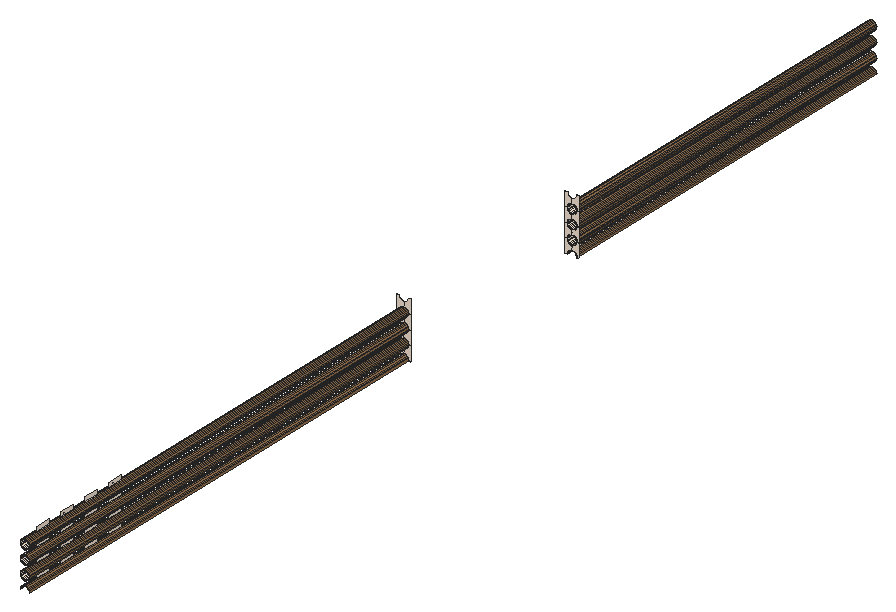
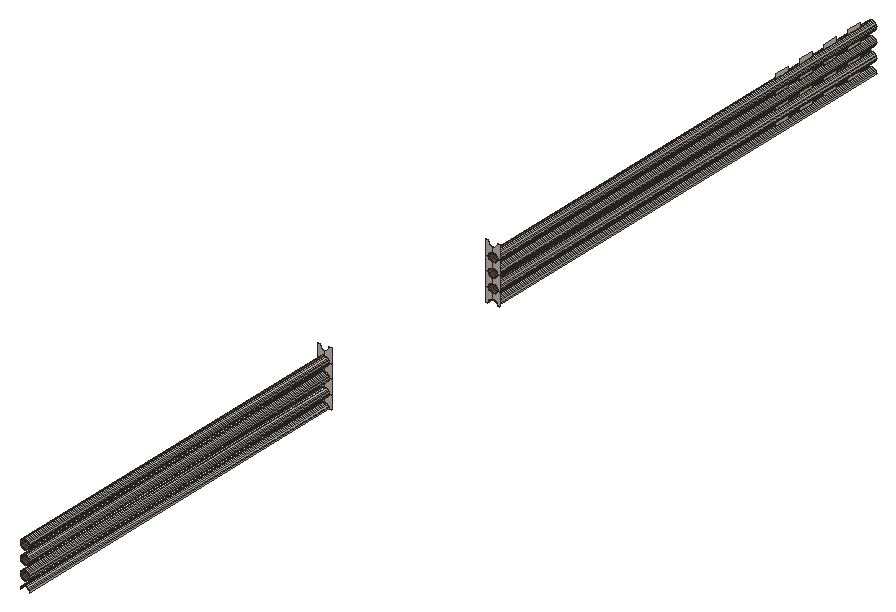
# SketchUp Ruby script. Lengths in inches.
U = 1.inch
M = Sketchup.active_model
def pt(a) = Geom::Point3d.new(a.map { |v| v * U })
def face(e, loops, mat)
  f = e.add_face(loops[0].map { |a| pt(a) })
  loops[1..].each { |l| e.add_face(l.map { |a| pt(a) }).erase! }
  f.material = f.back_material = mat if mat
  f
end
# faces: each face lists its corners as indices into pts; further lists are holes
def faces(e, pts, list, mat = nil) = list.each { |f| face(e, (f[0].is_a?(Array) ? f : [f]).map { |l| l.map { |i| pts[i] } }, mat) }
# xy, xz, yz: faces in a plane at the given z, y or x. An outline is a flat list of corners, or four numbers for a rectangle; further outlines are holes
def ring(l) = l.size == 4 ? [[l[0], l[1]], [l[2], l[1]], [l[2], l[3]], [l[0], l[3]]] : l.each_slice(2).to_a
def flat(e, list, mat, &to3) = list.each { |f| face(e, (f[0].is_a?(Array) ? f : [f]).map { |l| ring(l).map { |u, v| to3.(u, v) } }, mat) }
def xy(e, z, list, mat = nil) = flat(e, list, mat) { |x, y| [x, y, z] }
def xz(e, y, list, mat = nil) = flat(e, list, mat) { |x, z| [x, y, z] }
def yz(e, x, list, mat = nil) = flat(e, list, mat) { |y, z| [x, y, z] }
def lines(e, pts, list) = list.each { |a, b| e.add_line(pt(pts[a]), pt(pts[b])) }
# prism: a flat outline (further loops are holes) pulled along v
def prism(e, loops, v, mat = nil)
  f = face(e, loops, mat); d = Geom::Vector3d.new(v.map { |x| x * U })
  f.pushpull(f.normal.samedirection?(d) ? d.length : -d.length)
end
def box(e, o, s, mat = nil) = prism(e, [[o, [o[0] + s[0], o[1], o[2]], [o[0] + s[0], o[1] + s[1], o[2]], [o[0], o[1] + s[1], o[2]]]], [0, 0, s[2]], mat)
def at(x, y, z, deg = 0) = Geom::Transformation.translation(pt([x, y, z])) * Geom::Transformation.rotation(ORIGIN, Z_AXIS, deg.degrees)
def axes(o, x, y, z) = Geom::Transformation.new([*x, 0, *y, 0, *z, 0, *pt(o).to_a, 1])
def part(name) = M.definitions.add(name)
# library, detail: a bought-in or finely detailed component or shape, given as its bounding box
def library(name, o, s) = part(name).tap { |d| box(d.entities, o, s) }
def detail(e, o, s) = box(e.add_group.entities, o, s)
def put(e, d, t, mat = nil) = e.add_instance(d, t).tap { |i| i.material = mat if mat }
def group(e, t, mat = nil) = e.add_group.tap { |g| g.transformation = t; g.material = mat if mat }.entities
root = M.entities
M.materials.add("C01_Vanilla_Cream").color = [244, 228, 212]
M.materials.add("Wood_Floor_01_1K").color = [146, 111, 76]
xz(root,216,[[354,168,355,168,355.07,168.52,355.27,169,355.59,169.41,356,169.73,356.48,169.93,357,170,357,172,356.48,172.07,356,172.27,355.59,172.59,355.27,173,355.07,173.48,355,174,354,174],[359,168,360,168,360,174,359,174,358.93,173.48,358.73,173,358.41,172.59,358,172.27,357.52,172.07,357,172,357,170,357.52,169.93,358,169.73,358.41,169.41,358.73,169,358.93,168.52],[354,174,355,174,355.07,174.52,355.27,175,355.59,175.41,356,175.73,356.48,175.93,357,176,357,178,356.48,178.07,356,178.27,355.59,178.59,355.27,179,355.07,179.48,355,180,354,180],[359,174,360,174,360,180,359,180,358.93,179.48,358.73,179,358.41,178.59,358,178.27,357.52,178.07,357,178,357,176,357.52,175.93,358,175.73,358.41,175.41,358.73,175,358.93,174.52],[354,180,355,180,355.07,180.52,355.27,181,355.59,181.41,356,181.73,356.48,181.93,357,182,357,184,356.48,184.07,356,184.27,355.59,184.59,355.27,185,355.07,185.48,355,186,354,186],
  [359,180,360,180,360,186,359,186,358.93,185.48,358.73,185,358.41,184.59,358,184.27,357.52,184.07,357,184,357,182,357.52,181.93,358,181.73,358.41,181.41,358.73,181,358.93,180.52],[354,186,355,186,355.07,186.52,355.27,187,355.59,187.41,356,187.73,356.48,187.93,357,188,357,190,356.48,190.07,356,190.27,355.59,190.59,355.27,191,355.07,191.48,355,192,354,192],[359,186,360,186,360,192,359,192,358.93,191.48,358.73,191,358.41,190.59,358,190.27,357.52,190.07,357,190,357,188,357.52,187.93,358,187.73,358.41,187.41,358.73,187,358.93,186.52]],"C01_Vanilla_Cream")
xz(root,306.76,[[354,168,354,174,355,174,355.07,173.48,355.27,173,355.59,172.59,356,172.27,356.48,172.07,357,172,357,170,356.48,169.93,356,169.73,355.59,169.41,355.27,169,355.07,168.52,355,168],[359,168,358.93,168.52,358.73,169,358.41,169.41,358,169.73,357.52,169.93,357,170,357,172,357.52,172.07,358,172.27,358.41,172.59,358.73,173,358.93,173.48,359,174,360,174,360,168],[354,174,354,180,355,180,355.07,179.48,355.27,179,355.59,178.59,356,178.27,356.48,178.07,357,178,357,176,356.48,175.93,356,175.73,355.59,175.41,355.27,175,355.07,174.52,355,174],[359,174,358.93,174.52,358.73,175,358.41,175.41,358,175.73,357.52,175.93,357,176,357,178,357.52,178.07,358,178.27,358.41,178.59,358.73,179,358.93,179.48,359,180,360,180,360,174],[354,180,354,186,355,186,355.07,185.48,355.27,185,355.59,184.59,356,184.27,356.48,184.07,357,184,357,182,356.48,181.93,356,181.73,355.59,181.41,355.27,181,355.07,180.52,355,180],
  [359,180,358.93,180.52,358.73,181,358.41,181.41,358,181.73,357.52,181.93,357,182,357,184,357.52,184.07,358,184.27,358.41,184.59,358.73,185,358.93,185.48,359,186,360,186,360,180],[354,186,354,192,355,192,355.07,191.48,355.27,191,355.59,190.59,356,190.27,356.48,190.07,357,190,357,188,356.48,187.93,356,187.73,355.59,187.41,355.27,187,355.07,186.52,355,186],[359,186,358.93,186.52,358.73,187,358.41,187.41,358,187.73,357.52,187.93,357,188,357,190,357.52,190.07,358,190.27,358.41,190.59,358.73,191,358.93,191.48,359,192,360,192,360,186]],"C01_Vanilla_Cream")
yz(root,357,[[18.46,170,24.91,172],[31.37,170,37.83,172],[44.28,170,50.74,172],[57.2,170,63.65,172],[18.46,172,24.91,176],
  [31.37,172,37.83,176],[44.28,172,50.74,176],[57.2,172,63.65,176],[18.46,176,24.91,178],[31.37,176,37.83,178],
  [44.28,176,50.74,178],[57.2,176,63.65,178],[18.46,178,24.91,182],[31.37,178,37.83,182],[44.28,178,50.74,182],
  [57.2,178,63.65,182],[18.46,182,24.91,184],[31.37,182,37.83,184],[44.28,182,50.74,184],[57.2,182,63.65,184],
  [18.46,184,24.91,188],[31.37,184,37.83,188],[44.28,184,50.74,188],[57.2,184,63.65,188],[18.46,188,24.91,190],
  [31.37,188,37.83,190],[44.28,188,50.74,190],[57.2,188,63.65,190]],"C01_Vanilla_Cream")
p = [[355.07,216,168.52],[355,216,168],[355,12,168],[355.07,12,168.52],[359,216,168],[358.93,216,168.52],
  [358.93,12,168.52],[359,12,168],[355,306.76,168],[355.07,306.76,168.52],[355.07,468,168.52],[355,468,168],
  [358.93,306.76,168.52],[359,306.76,168],[359,468,168],[358.93,468,168.52],[355.27,216,169],[355.27,12,169],
  [358.73,216,169],[358.73,12,169],[355.27,306.76,169],[355.27,468,169],[358.73,306.76,169],[358.73,468,169],
  [355.59,216,169.41],[355.59,12,169.41],[358.41,216,169.41],[358.41,12,169.41],[355.59,306.76,169.41],[355.59,468,169.41],
  [358.41,306.76,169.41],[358.41,468,169.41],[356,216,169.73],[356,12,169.73],[358,216,169.73],[358,12,169.73],
  [356,306.76,169.73],[356,468,169.73],[358,306.76,169.73],[358,468,169.73],[356.48,216,169.93],[356.48,12,169.93],
  [357.52,216,169.93],[357.52,12,169.93],[356.48,306.76,169.93],[356.48,468,169.93],[357.52,306.76,169.93],[357.52,468,169.93],
  [357,216,170],[357,12,170],[357,18.46,170],[357,24.91,170],[357,31.37,170],[357,37.83,170],
  [357,44.28,170],[357,50.74,170],[357,57.2,170],[357,63.65,170],[357,306.76,170],[357,468,170],
  [356.48,216,172.07],[357,216,172],[357,63.65,172],[357,57.2,172],[357,50.74,172],[357,44.28,172],
  [357,37.83,172],[357,31.37,172],[357,24.91,172],[357,18.46,172],[357,12,172],[356.48,12,172.07],
  [357.52,216,172.07],[357.52,12,172.07],[357,306.76,172],[356.48,306.76,172.07],[356.48,468,172.07],[357,468,172],
  [357.52,306.76,172.07],[357.52,468,172.07],[356,216,172.27],[356,12,172.27],[358,216,172.27],[358,12,172.27],
  [356,306.76,172.27],[356,468,172.27],[358,306.76,172.27],[358,468,172.27],[355.59,216,172.59],[355.59,12,172.59],
  [358.41,216,172.59],[358.41,12,172.59],[355.59,306.76,172.59],[355.59,468,172.59],[358.41,306.76,172.59],[358.41,468,172.59],
  [355.27,216,173],[355.27,12,173],[358.73,216,173],[358.73,12,173],[355.27,306.76,173],[355.27,468,173],
  [358.73,306.76,173],[358.73,468,173],[355.07,216,173.48],[355.07,12,173.48],[358.93,216,173.48],[358.93,12,173.48],
  [355.07,306.76,173.48],[355.07,468,173.48],[358.93,306.76,173.48],[358.93,468,173.48],[355,216,174],[355,12,174],
  [359,216,174],[359,12,174],[355,306.76,174],[355,468,174],[359,306.76,174],[359,468,174],
  [355.07,216,174.52],[355.07,12,174.52],[358.93,216,174.52],[358.93,12,174.52],[355.07,306.76,174.52],[355.07,468,174.52],
  [358.93,306.76,174.52],[358.93,468,174.52],[355.27,216,175],[355.27,12,175],[358.73,216,175],[358.73,12,175],
  [355.27,306.76,175],[355.27,468,175],[358.73,306.76,175],[358.73,468,175],[355.59,216,175.41],[355.59,12,175.41],
  [358.41,216,175.41],[358.41,12,175.41],[355.59,306.76,175.41],[355.59,468,175.41],[358.41,306.76,175.41],[358.41,468,175.41],
  [356,216,175.73],[356,12,175.73],[358,216,175.73],[358,12,175.73],[356,306.76,175.73],[356,468,175.73],
  [358,306.76,175.73],[358,468,175.73],[356.48,216,175.93],[356.48,12,175.93],[357.52,216,175.93],[357.52,12,175.93],
  [356.48,306.76,175.93],[356.48,468,175.93],[357.52,306.76,175.93],[357.52,468,175.93],[357,216,176],[357,12,176],
  [357,18.46,176],[357,24.91,176],[357,31.37,176],[357,37.83,176],[357,44.28,176],[357,50.74,176],
  [357,57.2,176],[357,63.65,176],[357,306.76,176],[357,468,176],[356.48,216,178.07],[357,216,178],
  [357,63.65,178],[357,57.2,178],[357,50.74,178],[357,44.28,178],[357,37.83,178],[357,31.37,178],
  [357,24.91,178],[357,18.46,178],[357,12,178],[356.48,12,178.07],[357.52,216,178.07],[357.52,12,178.07],
  [357,306.76,178],[356.48,306.76,178.07],[356.48,468,178.07],[357,468,178],[357.52,306.76,178.07],[357.52,468,178.07],
  [356,216,178.27],[356,12,178.27],[358,216,178.27],[358,12,178.27],[356,306.76,178.27],[356,468,178.27],
  [358,306.76,178.27],[358,468,178.27],[355.59,216,178.59],[355.59,12,178.59],[358.41,216,178.59],[358.41,12,178.59],
  [355.59,306.76,178.59],[355.59,468,178.59],[358.41,306.76,178.59],[358.41,468,178.59],[355.27,216,179],[355.27,12,179],
  [358.73,216,179],[358.73,12,179],[355.27,306.76,179],[355.27,468,179],[358.73,306.76,179],[358.73,468,179],
  [355.07,216,179.48],[355.07,12,179.48],[358.93,216,179.48],[358.93,12,179.48],[355.07,306.76,179.48],[355.07,468,179.48],
  [358.93,306.76,179.48],[358.93,468,179.48],[355,216,180],[355,12,180],[359,216,180],[359,12,180],
  [355,306.76,180],[355,468,180],[359,306.76,180],[359,468,180],[355.07,216,180.52],[355.07,12,180.52],
  [358.93,216,180.52],[358.93,12,180.52],[355.07,306.76,180.52],[355.07,468,180.52],[358.93,306.76,180.52],[358.93,468,180.52],
  [355.27,216,181],[355.27,12,181],[358.73,216,181],[358.73,12,181],[355.27,306.76,181],[355.27,468,181],
  [358.73,306.76,181],[358.73,468,181],[355.59,216,181.41],[355.59,12,181.41],[358.41,216,181.41],[358.41,12,181.41],
  [355.59,306.76,181.41],[355.59,468,181.41],[358.41,306.76,181.41],[358.41,468,181.41],[356,216,181.73],[356,12,181.73],
  [358,216,181.73],[358,12,181.73],[356,306.76,181.73],[356,468,181.73],[358,306.76,181.73],[358,468,181.73],
  [356.48,216,181.93],[356.48,12,181.93],[357.52,216,181.93],[357.52,12,181.93],[356.48,306.76,181.93],[356.48,468,181.93],
  [357.52,306.76,181.93],[357.52,468,181.93],[357,216,182],[357,12,182],[357,18.46,182],[357,24.91,182],
  [357,31.37,182],[357,37.83,182],[357,44.28,182],[357,50.74,182],[357,57.2,182],[357,63.65,182],
  [357,306.76,182],[357,468,182],[356.48,216,184.07],[357,216,184],[357,63.65,184],[357,57.2,184],
  [357,50.74,184],[357,44.28,184],[357,37.83,184],[357,31.37,184],[357,24.91,184],[357,18.46,184],
  [357,12,184],[356.48,12,184.07],[357.52,216,184.07],[357.52,12,184.07],[357,306.76,184],[356.48,306.76,184.07],
  [356.48,468,184.07],[357,468,184],[357.52,306.76,184.07],[357.52,468,184.07],[356,216,184.27],[356,12,184.27],
  [358,216,184.27],[358,12,184.27],[356,306.76,184.27],[356,468,184.27],[358,306.76,184.27],[358,468,184.27],
  [355.59,216,184.59],[355.59,12,184.59],[358.41,216,184.59],[358.41,12,184.59],[355.59,306.76,184.59],[355.59,468,184.59],
  [358.41,306.76,184.59],[358.41,468,184.59],[355.27,216,185],[355.27,12,185],[358.73,216,185],[358.73,12,185],
  [355.27,306.76,185],[355.27,468,185],[358.73,306.76,185],[358.73,468,185],[355.07,216,185.48],[355.07,12,185.48],
  [358.93,216,185.48],[358.93,12,185.48],[355.07,306.76,185.48],[355.07,468,185.48],[358.93,306.76,185.48],[358.93,468,185.48],
  [355,216,186],[355,12,186],[359,216,186],[359,12,186],[355,306.76,186],[355,468,186],
  [359,306.76,186],[359,468,186],[355.07,216,186.52],[355.07,12,186.52],[358.93,216,186.52],[358.93,12,186.52],
  [355.07,306.76,186.52],[355.07,468,186.52],[358.93,306.76,186.52],[358.93,468,186.52],[355.27,216,187],[355.27,12,187],
  [358.73,216,187],[358.73,12,187],[355.27,306.76,187],[355.27,468,187],[358.73,306.76,187],[358.73,468,187],
  [355.59,216,187.41],[355.59,12,187.41],[358.41,216,187.41],[358.41,12,187.41],[355.59,306.76,187.41],[355.59,468,187.41],
  [358.41,306.76,187.41],[358.41,468,187.41],[356,216,187.73],[356,12,187.73],[358,216,187.73],[358,12,187.73],
  [356,306.76,187.73],[356,468,187.73],[358,306.76,187.73],[358,468,187.73],[356.48,216,187.93],[356.48,12,187.93],
  [357.52,216,187.93],[357.52,12,187.93],[356.48,306.76,187.93],[356.48,468,187.93],[357.52,306.76,187.93],[357.52,468,187.93],
  [357,216,188],[357,12,188],[357,18.46,188],[357,24.91,188],[357,31.37,188],[357,37.83,188],
  [357,44.28,188],[357,50.74,188],[357,57.2,188],[357,63.65,188],[357,306.76,188],[357,468,188]]
faces(root,p,[[0,1,2,3],[8,9,10,11],[16,0,3,17],[9,20,21,10],[24,16,17,25],[20,28,29,21],[32,24,25,33],[28,36,37,29],
  [40,32,33,41],[36,44,45,37],[48,40,41,49,50,51,52,53,54,55,56,57],[44,58,59,45],[60,61,62,63,64,65,66,67,68,69,70,71],[74,75,76,77],[80,60,71,81],[75,84,85,76],
  [88,80,81,89],[84,92,93,85],[96,88,89,97],[92,100,101,93],[104,96,97,105],[100,108,109,101],[112,104,105,113],[108,116,117,109],
  [120,112,113,121],[116,124,125,117],[128,120,121,129],[124,132,133,125],[136,128,129,137],[132,140,141,133],[144,136,137,145],[140,148,149,141],
  [152,144,145,153],[148,156,157,149],[160,152,153,161,162,163,164,165,166,167,168,169],[156,170,171,157],[172,173,174,175,176,177,178,179,180,181,182,183],[186,187,188,189],[192,172,183,193],[187,196,197,188],
  [200,192,193,201],[196,204,205,197],[208,200,201,209],[204,212,213,205],[216,208,209,217],[212,220,221,213],[224,216,217,225],[220,228,229,221],
  [232,224,225,233],[228,236,237,229],[240,232,233,241],[236,244,245,237],[248,240,241,249],[244,252,253,245],[256,248,249,257],[252,260,261,253],
  [264,256,257,265],[260,268,269,261],[272,264,265,273,274,275,276,277,278,279,280,281],[268,282,283,269],[284,285,286,287,288,289,290,291,292,293,294,295],[298,299,300,301],[304,284,295,305],[299,308,309,300],
  [312,304,305,313],[308,316,317,309],[320,312,313,321],[316,324,325,317],[328,320,321,329],[324,332,333,325],[336,328,329,337],[332,340,341,333],
  [344,336,337,345],[340,348,349,341],[352,344,345,353],[348,356,357,349],[360,352,353,361],[356,364,365,357],[368,360,361,369],[364,372,373,365],
  [376,368,369,377],[372,380,381,373],[384,376,377,385,386,387,388,389,390,391,392,393],[380,394,395,381]],"C01_Vanilla_Cream")
faces(root,p,[[4,5,6,7],[12,13,14,15],[5,18,19,6],[22,12,15,23],[18,26,27,19],[30,22,23,31],[26,34,35,27],[38,30,31,39],
  [34,42,43,35],[46,38,39,47],[42,48,57,56,55,54,53,52,51,50,49,43],[58,46,47,59],[61,72,73,70,69,68,67,66,65,64,63,62],[78,74,77,79],[72,82,83,73],[86,78,79,87],
  [82,90,91,83],[94,86,87,95],[90,98,99,91],[102,94,95,103],[98,106,107,99],[110,102,103,111],[106,114,115,107],[118,110,111,119],
  [114,122,123,115],[126,118,119,127],[122,130,131,123],[134,126,127,135],[130,138,139,131],[142,134,135,143],[138,146,147,139],[150,142,143,151],
  [146,154,155,147],[158,150,151,159],[154,160,169,168,167,166,165,164,163,162,161,155],[170,158,159,171],[173,184,185,182,181,180,179,178,177,176,175,174],[190,186,189,191],[184,194,195,185],[198,190,191,199],
  [194,202,203,195],[206,198,199,207],[202,210,211,203],[214,206,207,215],[210,218,219,211],[222,214,215,223],[218,226,227,219],[230,222,223,231],
  [226,234,235,227],[238,230,231,239],[234,242,243,235],[246,238,239,247],[242,250,251,243],[254,246,247,255],[250,258,259,251],[262,254,255,263],
  [258,266,267,259],[270,262,263,271],[266,272,281,280,279,278,277,276,275,274,273,267],[282,270,271,283],[285,296,297,294,293,292,291,290,289,288,287,286],[302,298,301,303],[296,306,307,297],[310,302,303,311],
  [306,314,315,307],[318,310,311,319],[314,322,323,315],[326,318,319,327],[322,330,331,323],[334,326,327,335],[330,338,339,331],[342,334,335,343],
  [338,346,347,339],[350,342,343,351],[346,354,355,347],[358,350,351,359],[354,362,363,355],[366,358,359,367],[362,370,371,363],[374,366,367,375],
  [370,378,379,371],[382,374,375,383],[378,384,393,392,391,390,389,388,387,386,385,379],[394,382,383,395]],"Wood_Floor_01_1K")
